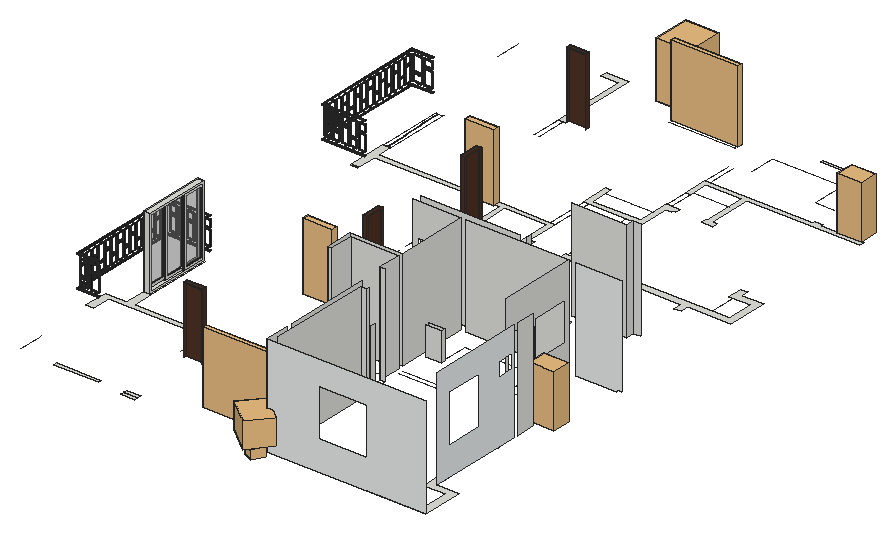
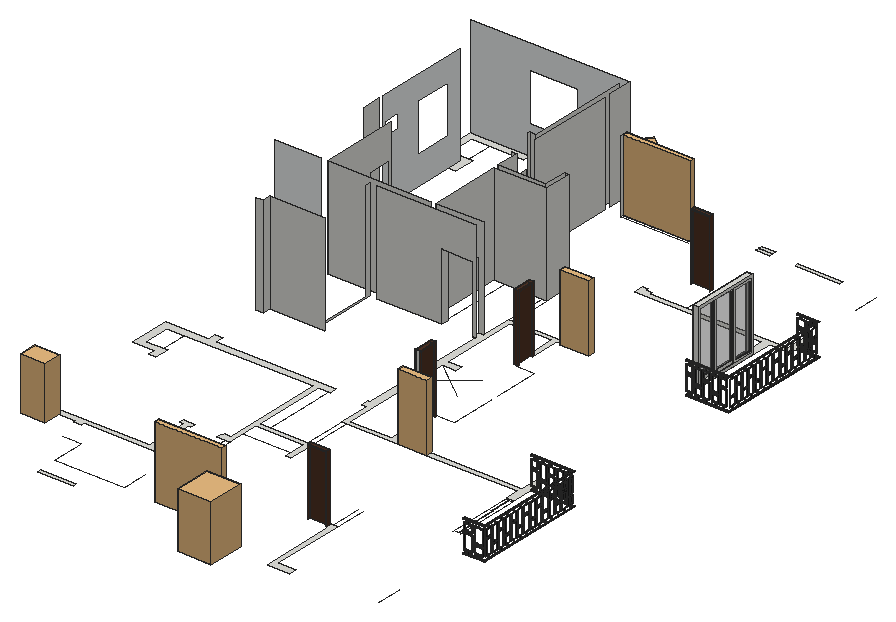
# SketchUp Ruby script. Lengths in inches.
U = 1.inch
M = Sketchup.active_model
def pt(a) = Geom::Point3d.new(a.map { |v| v * U })
def face(e, loops, mat)
  f = e.add_face(loops[0].map { |a| pt(a) })
  loops[1..].each { |l| e.add_face(l.map { |a| pt(a) }).erase! }
  f.material = f.back_material = mat if mat
  f
end
# faces: each face lists its corners as indices into pts; further lists are holes
def faces(e, pts, list, mat = nil) = list.each { |f| face(e, (f[0].is_a?(Array) ? f : [f]).map { |l| l.map { |i| pts[i] } }, mat) }
# xy, xz, yz: faces in a plane at the given z, y or x. An outline is a flat list of corners, or four numbers for a rectangle; further outlines are holes
def ring(l) = l.size == 4 ? [[l[0], l[1]], [l[2], l[1]], [l[2], l[3]], [l[0], l[3]]] : l.each_slice(2).to_a
def flat(e, list, mat, &to3) = list.each { |f| face(e, (f[0].is_a?(Array) ? f : [f]).map { |l| ring(l).map { |u, v| to3.(u, v) } }, mat) }
def xy(e, z, list, mat = nil) = flat(e, list, mat) { |x, y| [x, y, z] }
def xz(e, y, list, mat = nil) = flat(e, list, mat) { |x, z| [x, y, z] }
def yz(e, x, list, mat = nil) = flat(e, list, mat) { |y, z| [x, y, z] }
def lines(e, pts, list) = list.each { |a, b| e.add_line(pt(pts[a]), pt(pts[b])) }
# prism: a flat outline (further loops are holes) pulled along v
def prism(e, loops, v, mat = nil)
  f = face(e, loops, mat); d = Geom::Vector3d.new(v.map { |x| x * U })
  f.pushpull(f.normal.samedirection?(d) ? d.length : -d.length)
end
def box(e, o, s, mat = nil) = prism(e, [[o, [o[0] + s[0], o[1], o[2]], [o[0] + s[0], o[1] + s[1], o[2]], [o[0], o[1] + s[1], o[2]]]], [0, 0, s[2]], mat)
def at(x, y, z, deg = 0) = Geom::Transformation.translation(pt([x, y, z])) * Geom::Transformation.rotation(ORIGIN, Z_AXIS, deg.degrees)
def axes(o, x, y, z) = Geom::Transformation.new([*x, 0, *y, 0, *z, 0, *pt(o).to_a, 1])
def part(name) = M.definitions.add(name)
# library, detail: a bought-in or finely detailed component or shape, given as its bounding box
def library(name, o, s) = part(name).tap { |d| box(d.entities, o, s) }
def detail(e, o, s) = box(e.add_group.entities, o, s)
def put(e, d, t, mat = nil) = e.add_instance(d, t).tap { |i| i.material = mat if mat }
def group(e, t, mat = nil) = e.add_group.tap { |g| g.transformation = t; g.material = mat if mat }.entities
root = M.entities
M.materials.add("02 - Default").color = [196, 209, 187]
M.materials.add("02 - DefaultW").color = [91, 118, 29]
M.materials.add("04 - Default").color = [38, 38, 38]
M.materials.add("04 - DefaultW").color = [92, 55, 26]
M.materials.add("06 - Default").color = [255, 255, 255]
M.materials.add("07 - Default").color = [92, 55, 26]
M.materials.add("10 - Default").color = [62, 56, 39]
M.materials.add("Polis06_194").color = [79, 50, 36]
M.materials.add("[3P0081_White-City]").color = [235, 238, 238]
M.materials.add("[Color M00]").color = [255, 255, 255]
M.materials.add("[Color M08]").color = [30, 30, 30]
M.materials.add("[Translucent Glass Gray]").color = [128, 128, 128]
M.materials["[Translucent Glass Gray]"].alpha = 0.5
c1 = library("MONSTERA_Defintion",[-100.72,-132.16,0],[226.75,232.88,1000])
c2 = library("MONSTERA_Defintion1",[-382.23,-503.1,29.34],[811.96,1000,773.77])
c3 = library("POT_Defintion",[-467.71,-467.71,0],[935.42,935.42,1000])
c4 = library("POT_Defintion6",[-504.36,-499.05,1069.94],[1000,1000,51.81])
c5 = library("TABLE_Defintion5",[-349.98,-500,-99.29],[912.18,1000,162.92])
c6 = library("TABLE_Defintion3",[-282.7,-491.23,-690.5],[848.82,1000,669.35])
c7 = library("TABLE_Defintion",[-354.24,-500,-9.27],[914.7,1000,77.28])
c8 = part("Monstera Plant 50")
g1 = group(c8.entities,at(0,0,0))
g2 = group(g1,at(0,0,0))
put(g2,c1,axes([-70.21,316.62,1332.52],[0.60525,0.72131,0],[-0.72131,0.60525,0],[0,0,0.92363]),"02 - DefaultW")
put(g2,c2,axes([-70.21,316.62,1332.52],[2.09136,2.49238,0],[-2.49238,2.09136,0],[0,0,3.1915]),"02 - Default")
g3 = group(c8.entities,at(0,0,0))
g4 = group(g3,at(0,0,0))
put(g4,c3,axes([-63.73,311.08,962.21],[0.47902,0.57088,0],[-0.57088,0.47902,0],[0,0,0.69328]),"04 - Default")
put(g4,c4,axes([-63.73,311.08,962.21],[0.41695,0.4969,0],[-0.4969,0.41695,0],[0,0,0.60345]),"10 - Default")
g5 = group(c8.entities,at(0,0,0))
g6 = group(g5,at(0,0,0))
put(g6,c5,axes([-8.95,303.3125,886.6],[1.07163,-0.6187,0],[0.6187,1.07163,0],[0,0,1.23741]),"04 - DefaultW")
put(g6,c6,axes([-8.95,303.3125,886.6],[1.11435,-0.64337,0],[0.64337,1.11435,0],[0,0,1.28674]),"07 - Default")
put(g6,c7,axes([-8.95,303.3125,886.6],[1.10303,-0.63684,0],[0.63684,1.10303,0],[0,0,1.27367]),"06 - Default")
c9 = library("cay+chuoi",[26.89,19.66,0.52],[41.96,45.65,69.71])
c10 = library("Scara cu plante",[-7.66,-9.41,-0.15],[30.59,22.83,66.38])
c11 = part("Group\#70")
prism(c11.entities,[[[4.13,0,3.9375],[7.875,0,3.9375],[7.875,0,13.78],[4.13,0,13.78],[4.13,0,15.75],[7.875,0,15.75],[7.875,0,35.43],[4.13,0,35.43],[4.13,0,39.37],[3.74,0,39.37],[3.74,0,35.43],[0,0,35.43],[0,0,15.75],[3.74,0,15.75],[3.74,0,13.78],[0,0,13.78],[0,0,3.9375],[3.74,0,3.9375],[3.74,0,0],[4.13,0,0]],[[0.39,0,16.14],[0.39,0,35.04],[7.48,0,35.04],[7.48,0,16.14]],[[7.48,0,4.33],[0.39,0,4.33],[0.39,0,13.39],[7.48,0,13.39]]],[0,0.39,0],"[Color M08]")
c12 = part("Group\#69")
prism(c12.entities,[[[3.74,0,35.43],[0,0,35.43],[0,0,25.59],[3.74,0,25.59],[3.74,0,23.62],[0,0,23.62],[0,0,3.9375],[3.74,0,3.9375],[3.74,0,0],[4.13,0,0],[4.13,0,3.9375],[7.875,0,3.9375],[7.875,0,23.62],[4.13,0,23.62],[4.13,0,25.59],[7.875,0,25.59],[7.875,0,35.43],[4.13,0,35.43],[4.13,0,39.37],[3.74,0,39.37]],[[7.48,0,23.23],[7.48,0,4.33],[0.39,0,4.33],[0.39,0,23.23]],[[0.39,0,35.04],[7.48,0,35.04],[7.48,0,25.98],[0.39,0,25.98]]],[0,0.39,0],"[Color M08]")
c13 = part("Group\#75")
put(c13.entities,c11,at(0,0,0))
put(c13.entities,c12,at(9.84,0,0))
c14 = part("Group\#76")
put(c14.entities,c11,at(0,0,0))
put(c14.entities,c12,at(9.84,0,0))
c15 = part("Group\#71")
put(c15.entities,c11,at(0,0,0))
put(c15.entities,c12,at(9.84,0,0))
c16 = part("Group\#74")
put(c16.entities,c13,axes([0.79,60.04,0.79],[0,1,0],[1,0,0],[0,0,1]))
put(c16.entities,c13,axes([0.79,40.35,0.79],[0,1,0],[1,0,0],[0,0,1]))
put(c16.entities,c13,axes([0.79,79.72,0.79],[0,1,0],[1,0,0],[0,0,1]))
g7 = group(c16.entities,at(0,0,40.16))
prism(g7,[[[54,-20.92,0],[0,-20.92,0],[0,120.08,0],[27,120.08,0],[27,118.11,0],[1.97,118.11,0],[1.97,-18.98,0],[54,-18.98,0]]],[0,0,0.79],"[Color M08]")
put(c16.entities,c14,axes([0.79,0.98,0.79],[0,1,0],[1,0,0],[0,0,1]))
put(c16.entities,c13,axes([0.79,20.67,0.79],[0,1,0],[1,0,0],[0,0,1]))
put(c16.entities,c13,axes([2.95,118.9,0.79],[1.35733,0,0],[0,1,0],[0,0,1]))
g8 = group(c16.entities,at(0,0,0))
prism(g8,[[[54,-20.92,0],[0,-20.92,0],[0,120.08,0],[27,120.08,0],[27,118.11,0],[1.97,118.11,0],[1.97,-18.98,0],[54,-18.98,0]]],[0,0,0.79],"[Color M08]")
put(c16.entities,c15,axes([0.79,99.41,0.79],[0,1,0],[1,0,0],[0,0,1]))
put(c16.entities,c14,axes([0.79,-18.7,0.79],[0,1,0],[1,0,0],[0,0,1]))
put(c16.entities,c14,axes([22.01,-20.17,0.79],[-1,0,0],[0,1,0],[0,0,1]))
g9 = group(c16.entities,at(43.22,-20.17,0.79))
put(g9,c11,axes([0,0,0],[-1,0,0],[0,1,0],[0,0,1]))
put(g9,c12,axes([-9.84,0,0],[-1,0,0],[0,1,0],[0,0,1]))
put(g9,c12,axes([10.78,0,0],[-1,0,0],[0,1,0],[0,0,1]))
c17 = part("Flush door")
xy(c17.entities,0,[[0,0,4.72,1.18],[0,34.25,4.72,35.43]],"Polis06_194")
xy(c17.entities,85.26,[[0,1.18,4.72,34.25]],"Polis06_194")
xy(c17.entities,86.61,[[0,0,4.72,35.43]],"Polis06_194")
xz(c17.entities,0,[[0,0,4.72,86.61]],"Polis06_194")
xz(c17.entities,1.18,[[0,0,2.36,85.26],[2.36,0,4.72,85.26]],"Polis06_194")
xz(c17.entities,34.25,[[0,0,4.72,85.26]],"Polis06_194")
xz(c17.entities,35.43,[[0,0,4.72,86.61]],"Polis06_194")
yz(c17.entities,0,[[0,0,1.18,86.61],[34.25,0,35.43,86.61],[1.18,85.26,34.25,86.61]],"Polis06_194")
yz(c17.entities,2.36,[[1.18,0,34.25,0,34.25,85.21,1.18,85.26]],"Polis06_194")
yz(c17.entities,4.72,[[0,0,1.18,86.61],[34.25,0,35.43,86.61],[1.18,85.26,34.25,86.61]],"Polis06_194")
c18 = part("구성 요소\#2")
prism(c18.entities,[[[0,0,0],[118.11,0,0],[118.11,0,78.74],[0,0,78.74]],[[116.14,0,76.77],[116.14,0,1.97],[1.97,0,1.97],[1.97,0,76.77]]],[0,7.875,0])
c19 = part("구성 요소\#1")
xy(c19.entities,0,[[[0,0,40.16,74.8],[2.375,2.375,37.78,72.43]]])
xy(c19.entities,1.18,[[2.375,2.375,37.78,72.43]],"[Translucent Glass Gray]")
xy(c19.entities,2.36,[[[0,0,40.16,74.8],[2.375,2.375,37.78,72.43]]])
xz(c19.entities,0,[[0,0,40.16,2.36]],"[Color M00]")
xz(c19.entities,2.375,[[2.375,0,37.78,1.18],[2.375,1.18,37.78,2.36]])
xz(c19.entities,72.43,[[2.375,0,37.78,1.18],[2.375,1.18,37.78,2.36]])
xz(c19.entities,74.8,[[0,0,40.16,2.36]],"[Color M00]")
yz(c19.entities,0,[[0,0,74.8,2.36]])
yz(c19.entities,2.375,[[2.375,0,72.43,1.18],[2.375,1.18,72.43,2.36]])
yz(c19.entities,37.78,[[2.375,0,72.43,1.18],[2.375,1.18,72.43,2.36]])
yz(c19.entities,40.16,[[0,0,74.8,2.36]])
c20 = part("구성 요소\#3")
xy(c20.entities,0,[[0,0,40.16,2.36]],"[Color M00]")
xy(c20.entities,2.375,[[2.375,0,37.78,1.18],[2.375,1.18,37.78,2.36]])
xy(c20.entities,35.83,[[38.48,0,39.47,0.39]])
xy(c20.entities,35.83,[[38.48,1.97,39.47,2.36]],"[Color M00]")
xy(c20.entities,38.98,[[38.48,0,39.47,0.39]])
xy(c20.entities,38.98,[[38.48,1.97,39.47,2.36]],"[Color M00]")
xy(c20.entities,72.43,[[2.375,0,37.78,1.18],[2.375,1.18,37.78,2.36]])
xy(c20.entities,74.8,[[0,0,40.16,2.36]],"[Color M00]")
xz(c20.entities,0,[[[0,0,40.16,74.8],[2.375,2.375,37.78,72.43],[38.48,35.83,39.47,38.98]]])
xz(c20.entities,0.39,[[38.48,35.83,39.47,38.98]])
xz(c20.entities,1.18,[[2.375,2.375,37.78,72.43]],"[Translucent Glass Gray]")
xz(c20.entities,1.97,[[38.48,35.83,39.47,38.98]],"[Color M00]")
xz(c20.entities,2.36,[[[0,0,40.16,74.8],[2.375,2.375,37.78,72.43],[38.48,35.83,39.47,38.98]]])
yz(c20.entities,0,[[0,0,2.36,74.8]])
yz(c20.entities,2.375,[[0,2.375,1.18,72.43],[1.18,2.375,2.36,72.43]])
yz(c20.entities,37.78,[[0,2.375,1.18,72.43],[1.18,2.375,2.36,72.43]])
yz(c20.entities,38.48,[[0,35.83,0.39,38.98]])
yz(c20.entities,38.48,[[1.97,35.83,2.36,38.98]],"[Color M00]")
yz(c20.entities,39.47,[[0,35.83,0.39,38.98]])
yz(c20.entities,39.47,[[1.97,35.83,2.36,38.98]],"[Color M00]")
yz(c20.entities,40.16,[[0,0,2.36,74.8]])
c21 = part("구성 요소\#4")
put(c21.entities,c19,axes([37.78,4.72,0],[1,0,0],[0,0,1],[0,-1,0]))
put(c21.entities,c20,at(75.5625,0,0))
put(c21.entities,c19,axes([0,7.09,0],[1,0,0],[0,0,1],[0,-1,0]))
c22 = part("그룹\#1")
put(c22.entities,c18,axes([0,0,0],[1.04,0,0],[0,1,0],[0,0,1]))
put(c22.entities,c21,axes([1.97,0.39,1.97],[1.02677,0,0],[0,1,0],[0,0,1]))
c23 = part("sliding door")
put(c23.entities,c22,at(0,0,0))
c24 = library("SLIDING+GLASS+DOOR",[0,-0.75,0],[72,5.75,80])
c25 = library("PINTU 6 YA",[0,-0.6875,0],[35.83,8.07,80.71])
xy(root,132,[[308,357.97,325.5,361.97],[614.5,357.97,614.5,366.97,679.5,366.97,679.5,399.97,652.5,399.97,652.5,426.87,661.5,426.87,661.5,408.97,688.5,408.97,688.5,357.97],[220,362.97,276,366.97],[308,362.97,325.5,366.97],[171,474.87,171,504.97,198,504.97,198,530.97,207,530.97,207,504.97,366,504.97,366,492.97,360,492.97,360,495.97,352,495.97,352,498.97,180,498.97,180,474.87],
  [652.5,504.97,661.5,505.03],[652.5,505.03,661.5,507.03],[357,624.97,357,630.97,363,630.97,363,666.97,369,666.97,369,630.97,421.5,630.97,421.5,726.97,404.25,726.97,404.25,735.97,421.5,735.97,421.5,774.97,404.25,774.97,404.25,783.97,421.5,783.97,421.5,879.97,369,879.97,369,843.97,363,843.97,363,879.97,357,879.97,357,885.97,427.5,885.97,427.5,846.97,433.5,846.97,433.5,837.97,430.5,837.97,430.5,672.97,433.5,672.97,433.5,663.97,427.5,663.97,427.5,624.97],[622.5,827.97,622.5,837.97,472.5,837.97,472.5,846.97,487.5,846.97,487.5,938.47,421.5,938.47,421.5,972.97,427.5,972.97,427.5,944.47,487.5,944.47,487.5,984.97,504,984.97,504,978.97,501.5,978.97,501.5,975.97,493.5,975.97,493.5,846.97,676.5,846.97,676.5,879.97,649.5,879.97,649.5,897.97,658.5,897.97,658.5,888.97,685.5,888.97,685.5,837.97,631.5,837.97,631.5,827.97],[198,853.97,207,855.97],
  [198,855.97,198,903.97,207,903.97,207,885.97,321,885.97,321,879.97,207,879.97,207,855.97],[536,978.97,536,984.97,538.5,984.97,538.5,1038.97,493.5,1038.97,493.5,1014.97,487.5,1014.97,487.5,1044.97,622.5,1044.97,622.5,1047.97,631.5,1047.97,631.5,1044.97,685.5,1044.97,685.5,1038.97,544.5,1038.97,544.5,984.97,550.5,984.97,550.5,978.97],[300,1050.97,300,1143.97,278,1143.97,278,1152.97,306,1152.97,306,1056.97,309,1056.97,309,1050.97],[552.5,1143.97,596.5,1147.97]])
xz(root,357.97,[[[490.5,132,688.5,258],[554.5,168,614.5,228]]],"[3P0081_White-City]")
xz(root,495.97,[[496.5,132,504.5,258]])
xz(root,537.97,[[421.5,132,427.5,258],[487.5,132,493.5,258]])
xz(root,566.47,[[427.5,132,487.5,258]])
xz(root,572.47,[[421.5,132,487.5,258]])
xz(root,597.97,[[622.5,132,631.5,216]])
xz(root,600.97,[[493.5,132,513.5,168]])
xz(root,606.97,[[493.5,132,513.5,168]])
xz(root,663.97,[[427.5,132,433.5,132,433.5,216,472.5,216,472.5,132,487.5,132,487.5,258,427.5,258],[493.5,132,622.5,258]])
xz(root,663.97,[[631.5,132,682.5,132,682.5,134,688.5,134,688.5,258,631.5,258]],"[3P0081_White-City]")
xz(root,672.97,[[430.5,132,430.5,258,553.5,258,553.5,132,472.5,132,472.5,216,433.5,216,433.5,132]])
xz(root,753.97,[[553.5,132,622.5,258]])
xz(root,763.97,[[622.5,132,631.5,258]])
xz(root,843.97,[[363,132,369,216]])
yz(root,421.5,[[537.97,132,572.47,258]])
yz(root,427.5,[[537.97,132,566.47,258]])
yz(root,470.25,[[387.97,132,396.97,222]])
yz(root,472.5,[[663.97,132,672.97,216]])
yz(root,487.5,[[537.97,132,566.47,258],[572.47,132,663.97,258]])
yz(root,490.5,[[357.97,132,387.97,258],[396.97,132,504.97,258]])
yz(root,496.5,[[366.97,132,495.97,258]])
yz(root,504.5,[[495.97,132,498.97,258]])
yz(root,507,[[498.97,132,504.97,216]])
yz(root,513.5,[[600.97,132,606.97,168]])
yz(root,562.5,[[672.97,132,741.97,132,741.97,134,678.97,134,678.97,258,672.97,258]])
yz(root,622.5,[[[564.97,132,564.97,258,663.97,258,663.97,132,597.97,132,597.97,216,567.97,216,567.97,132],[609.97,168,657.97,216]],[753.97,132,763.97,258]])
yz(root,661.5,[[535,132,558.97,258]])
yz(root,661.5,[[[408.97,132,529,258],[426.87,168,474.87,228],[504.97,210,526.53,228]]],"[3P0081_White-City]")
p = [[144,635.47,132],[198,635.47,132],[511.5,1086.97,132],[511.5,1119.97,132],[487.5,964.47,132],[427.5,964.47,132],
  [474.5,938.47,132],[474.5,846.97,132],[598.5,1077.97,132],[598.5,1119.97,132],[654.5,846.97,132],[654.5,879.97,132],
  [175,1143.97,132],[175,1110.97,132],[538.5,1018.97,132],[493.5,1018.97,132],[201.5,587.47,132],[201.5,585.97,132],
  [198,530.97,132],[198,532.97,132],[200.5,612.97,132],[200.5,585.97,132],[207,614.97,132],[207,612.97,132],
  [201.5,558.97,132],[202.5,558.97,132],[198,612.97,132],[202.5,587.47,132],[207,532.97,132],[203.5,532.97,132],
  [406.25,391.97,132],[446.25,391.97,132],[470.25,387.97,132],[468.25,387.97,132],[388.25,1113.97,132],[388.25,1122.97,132],
  [388.25,387.97,132],[388.25,396.97,132],[446.25,392.97,132],[202.5,932.97,132],[202.5,931.97,132],[203.5,559.97,132],
  [427.25,392.97,132],[203.5,932.97,132],[622.5,1077.97,132],[421.5,624.97,132],[421.5,572.47,132],[598.5,597.97,132],
  [598.5,639.97,132],[202.5,559.97,132],[470.25,1113.97,132],[468.25,1113.97,132],[200.5,958.97,132],[201.5,958.97,132],
  [468.25,1119.97,132],[427.25,1119.97,132],[386.25,1122.97,132],[468.25,1122.97,132],[446.25,1117.97,132],[446.25,1118.97,132],
  [406.25,1117.97,132],[363,817.97,132],[341,817.97,132],[406.25,392.97,132],[406.25,1118.97,132],[468.25,393.97,132],
  [427.25,393.97,132],[200.5,985.97,132],[207,905.97,132],[203.5,905.97,132],[487.5,1080.97,132],[487.5,1044.97,132],
  [421.5,885.97,132],[421.5,938.47,132],[207,987.97,132],[207,985.97,132],[622.5,597.97,132],[300,1050.97,132],
  [300,1011.97,132],[198,985.97,132],[468.25,396.97,132],[201.5,960.47,132],[427.25,1118.97,132],[386.25,396.97,132],
  [201.5,931.97,132],[198,903.97,132],[198,905.97,132],[202.5,960.47,132],[306,1050.97,132],[306,1011.97,132],
  [493.5,1014.97,132],[493.5,984.97,132],[541.5,558.97,132],[493.5,558.97,132],[541.5,564.97,132],[493.5,564.97,132],
  [306,498.97,132],[306,459.97,132],[341,692.97,132],[363,692.97,132],[487.5,1014.97,132],[487.5,984.97,132],
  [341,759.97,132],[341,750.97,132],[493.5,1080.97,132],[493.5,1044.97,132],[487.5,537.97,132],[487.5,504.97,132],
  [511.5,606.97,132],[511.5,639.97,132],[300,498.97,132],[300,459.97,132],[427.5,624.97,132],[427.5,572.47,132],
  [427.5,885.97,132],[427.5,938.47,132],[421.5,774.97,132],[396.75,755.47,132],[493.5,537.97,132],[493.5,504.97,132],
  [372,774.97,132],[421.5,735.97,132],[372,735.97,132],[202.5,532.97,132],[468.25,392.97,132],[207,903.97,132],
  [207,530.97,132],[201.5,612.97,132],[201.5,985.97,132],[468.25,1118.97,132],[202.5,905.97,132],[386.25,387.97,132],
  [386.25,1113.97,132],[487.5,546.47,132],[427.5,546.47,132],[198,614.97,132],[470.25,1122.97,132],[198,987.97,132],
  [175,366.97,132],[175,399.97,132],[470.25,396.97,132],[657.5,366.97,132],[657.5,399.97,132],[474.5,572.47,132],
  [474.5,663.97,132]]
lines(root,p,[[0,1],[2,3],[4,5],[6,7],[8,9],[10,11],[12,13],[14,15],[16,17],[18,19],[20,21],[22,23],
  [24,25],[26,20],[21,17],[27,16],[28,29],[30,31],[32,33],[34,35],[36,37],[31,38],[39,40],[29,41],
  [42,38],[43,39],[8,44],[45,46],[47,48],[49,25],[50,51],[52,53],[54,55],[56,35],[57,54],[58,59],
  [60,58],[61,62],[63,30],[64,60],[65,66],[67,52],[68,69],[70,71],[72,73],[74,75],[47,76],[69,43],
  [77,78],[41,49],[79,67],[80,65],[81,53],[55,82],[82,59],[83,37],[84,40],[85,86],[87,81],[66,42],
  [88,89],[90,91],[92,93],[94,95],[96,97],[98,99],[100,101],[62,102],[103,98],[104,105],[106,107],[108,109],
  [48,109],[110,111],[112,113],[114,115],[116,117],[118,119],[120,117],[117,121],[117,122],[25,123],[23,28],[17,24],
  [42,63],[35,57],[51,34],[124,33],[39,87],[68,125],[28,126],[49,27],[127,23],[19,26],[20,127],[29,123],
  [123,19],[16,127],[37,80],[38,124],[67,128],[33,36],[86,79],[54,129],[129,51],[53,84],[82,64],[40,130],
  [81,128],[59,129],[65,124],[36,131],[130,86],[34,132],[75,68],[69,130],[133,134],[9,3],[26,135],[57,136],
  [79,137],[138,139],[80,140],[128,75],[141,142],[143,144]])
put(root,c8,axes([483.73,342.98,131.46],[0.01275,0,0],[0,0.01275,0],[0,0,0.01275]))
put(root,c9,at(323.18,1120.82,131.22))
put(root,c10,axes([660.01,578.41,132],[1,0,0],[0,-1,0],[0,0,1]))
put(root,c10,axes([660.01,1058.41,132],[1,0,0],[0,-1,0],[0,0,1]))
put(root,c16,axes([144,896.4,132],[1,0,0],[0,1,0],[0,0,0.97692]))
put(root,c16,axes([144,614.55,132],[1,0,0],[0,-1,0],[0,0,0.97692]))
put(root,c17,axes([367.72,690.97,132],[-1,0,0],[0,-0.67733,0],[0,0,0.96982]))
put(root,c17,axes([367.72,819.97,132],[-1,0,0],[0,0.67733,0],[0,0,0.96982]))
put(root,c17,axes([333,458.7,132],[0,-1,0],[-0.67733,0,0],[0,0,0.96982]))
put(root,c17,axes([333,1052.25,132],[0,1,0],[-0.67733,0,0],[0,0,0.96982]))
put(root,c23,axes([198,614.97,132],[0,-0.68385,0],[1,0,0],[0,0,1.143]))
put(root,c24,axes([386.25,387.97,132],[1.16667,0,0],[0,1,0],[0,0,1.125]))
put(root,c24,axes([386.25,1122.97,132],[1.16667,0,0],[0,-1,0],[0,0,1.125]))
put(root,c25,axes([321,625.66,132],[1.00475,0,0],[0,1,0],[0,0,1.04078]))
put(root,c25,axes([321,885.29,132],[1.00475,0,0],[0,-1,0],[0,0,1.04078]))
